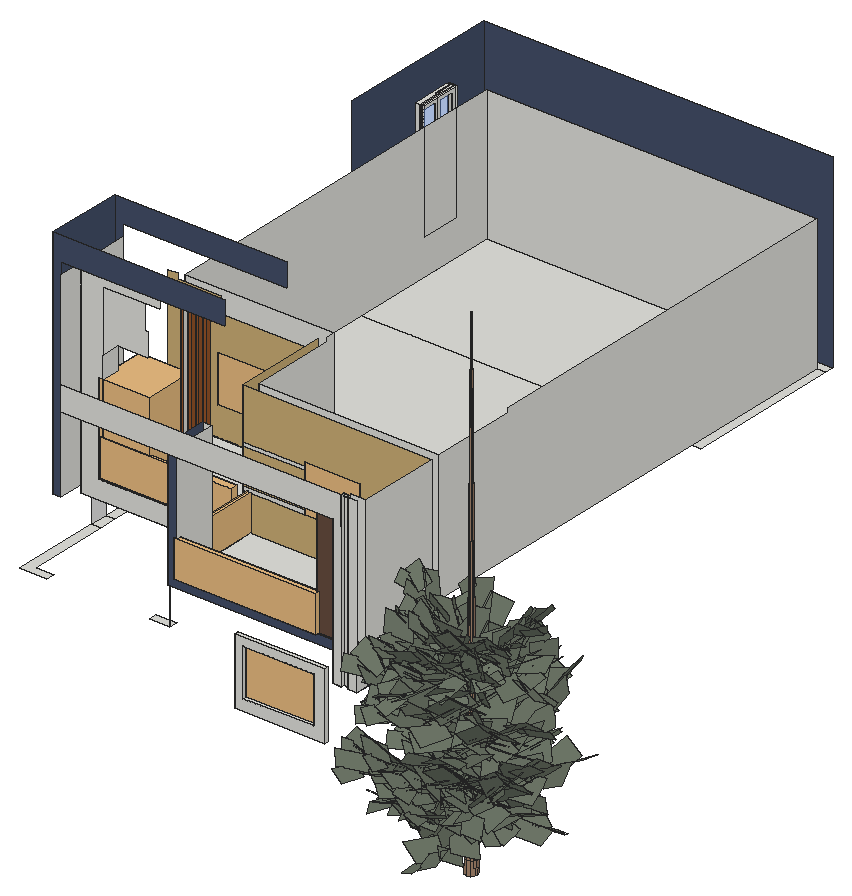
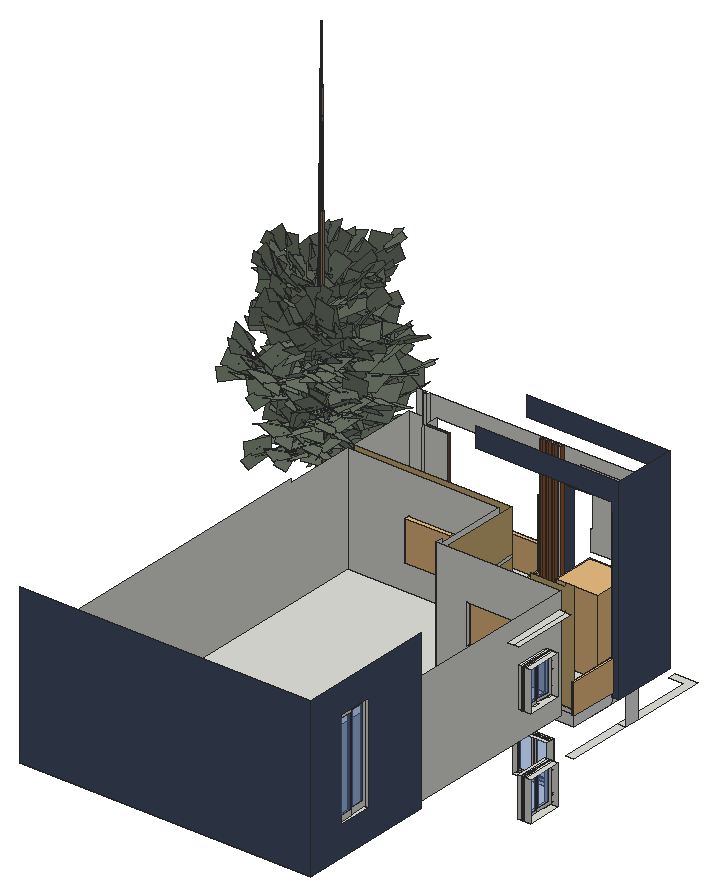
# SketchUp Ruby script. Lengths in inches.
U = 1.inch
M = Sketchup.active_model
def pt(a) = Geom::Point3d.new(a.map { |v| v * U })
def face(e, loops, mat)
  f = e.add_face(loops[0].map { |a| pt(a) })
  loops[1..].each { |l| e.add_face(l.map { |a| pt(a) }).erase! }
  f.material = f.back_material = mat if mat
  f
end
# faces: each face lists its corners as indices into pts; further lists are holes
def faces(e, pts, list, mat = nil) = list.each { |f| face(e, (f[0].is_a?(Array) ? f : [f]).map { |l| l.map { |i| pts[i] } }, mat) }
# xy, xz, yz: faces in a plane at the given z, y or x. An outline is a flat list of corners, or four numbers for a rectangle; further outlines are holes
def ring(l) = l.size == 4 ? [[l[0], l[1]], [l[2], l[1]], [l[2], l[3]], [l[0], l[3]]] : l.each_slice(2).to_a
def flat(e, list, mat, &to3) = list.each { |f| face(e, (f[0].is_a?(Array) ? f : [f]).map { |l| ring(l).map { |u, v| to3.(u, v) } }, mat) }
def xy(e, z, list, mat = nil) = flat(e, list, mat) { |x, y| [x, y, z] }
def xz(e, y, list, mat = nil) = flat(e, list, mat) { |x, z| [x, y, z] }
def yz(e, x, list, mat = nil) = flat(e, list, mat) { |y, z| [x, y, z] }
def lines(e, pts, list) = list.each { |a, b| e.add_line(pt(pts[a]), pt(pts[b])) }
# prism: a flat outline (further loops are holes) pulled along v
def prism(e, loops, v, mat = nil)
  f = face(e, loops, mat); d = Geom::Vector3d.new(v.map { |x| x * U })
  f.pushpull(f.normal.samedirection?(d) ? d.length : -d.length)
end
def box(e, o, s, mat = nil) = prism(e, [[o, [o[0] + s[0], o[1], o[2]], [o[0] + s[0], o[1] + s[1], o[2]], [o[0], o[1] + s[1], o[2]]]], [0, 0, s[2]], mat)
def at(x, y, z, deg = 0) = Geom::Transformation.translation(pt([x, y, z])) * Geom::Transformation.rotation(ORIGIN, Z_AXIS, deg.degrees)
def axes(o, x, y, z) = Geom::Transformation.new([*x, 0, *y, 0, *z, 0, *pt(o).to_a, 1])
def part(name) = M.definitions.add(name)
# library, detail: a bought-in or finely detailed component or shape, given as its bounding box
def library(name, o, s) = part(name).tap { |d| box(d.entities, o, s) }
def detail(e, o, s) = box(e.add_group.entities, o, s)
def put(e, d, t, mat = nil) = e.add_instance(d, t).tap { |i| i.material = mat if mat }
def group(e, t, mat = nil) = e.add_group.tap { |g| g.transformation = t; g.material = mat if mat }.entities
root = M.entities
M.materials.add("Marc_Shoes2").color = [68, 80, 105]
M.materials.add("Teddy_Glasses").color = [103, 77, 64]
M.materials.add("[Chipboard]").color = [205, 176, 119]
M.materials.add("[Translucent Glass Blue]").color = [100, 149, 237]
M.materials["[Translucent Glass Blue]"].alpha = 0.5
M.materials.add("[Wood Cherry Original]").color = [152, 86, 42]
M.materials.add("caule_pinheiro_fasdfa0d5asd9as0d15f9as16das5106w1560e1w6").color = [164, 132, 108]
M.materials.add("folha_pinheiro_fsadfaf0sa5f60a6s1d0fa19e01a601fw601").color = [111, 120, 105]
M.materials.add("white_wall").color = [233, 233, 233]
c1 = part("Janela aluminio")
xy(c1.entities,0,[[0,0,47.24,1.57],[23.62,1.57,47.24,2.76],[0,2.76,25.98,3.9375],[0,3.9375,47.24,5.91]])
xy(c1.entities,43.31,[[0,0,47.24,1.57],[23.62,1.57,47.24,2.76],[0,2.76,0,5.91,47.24,5.91,47.24,3.9375,25.98,3.9375,25.98,2.76],[25.98,2.76,47.24,3.9375]])
xz(c1.entities,1.57,[[0,0,23.62,0,23.62,41.34,21.26,41.34,21.26,1.97,1.97,1.97,1.97,41.34,23.62,41.34,23.62,43.31,0,43.31],[[23.62,0,47.24,43.31],[25.7,1.97,45.28,41.34]]])
xz(c1.entities,2.76,[[[0,0,23.62,43.31],[2.36,2.36,21.26,40.94]],[23.62,0,25.98,43.31]])
xz(c1.entities,2.76,[[2.36,2.36,21.26,40.94]],"[Translucent Glass Blue]")
xz(c1.entities,3.9375,[[25.98,0,25.98,2.36,44.88,2.36,44.88,40.94,25.98,40.94,25.98,43.31,47.24,43.31,47.24,0]])
xz(c1.entities,3.9375,[[25.98,2.36,44.88,40.94]],"[Translucent Glass Blue]")
yz(c1.entities,0,[[0,0,1.57,43.31],[2.76,0,5.91,43.31]])
yz(c1.entities,23.62,[[1.57,0,2.76,43.31]])
yz(c1.entities,25.98,[[2.76,0,3.9375,43.31]])
yz(c1.entities,47.24,[[0,0,1.57,43.31],[1.57,0,2.76,43.31],[3.9375,0,5.91,43.31]])
c2 = library("Janela+de+correr+1,50x1,00+m+VRAY",[0,0,0],[59.06,5.12,39.37])
c3 = part("bough01")
p = [[11.29,3.2,8.88],[13.41,4.42,-0.24],[13.19,18.86,1.64],[11.08,17.64,10.76],[8.3,5.16,4.77],[17.24,0,0],
  [26.01,15.19,0],[17.07,20.36,4.77],[7.28,2.65,0.91],[15.18,7.21,3.36],[7.9,19.82,3.36],[0,15.26,0.91],
  [8.87,11.62,4.48],[17.62,18.34,1.72],[8.85,32.26,7.82],[0.1,25.53,10.58],[10.83,18.83,5.84],[18.73,15.63,1.77],
  [26.01,27.18,6.84],[18.11,30.37,10.91],[8.25,26.54,5.5],[14.01,28.875,8.47],[10.03,38.73,8.47],[4.26,36.4,5.5],
  [10.04,24.31,6.06],[17.58,22.66,9.11],[19.2,35.07,11.83],[11.65,36.72,8.78]]
faces(c3.entities,p,[[0,1,2,3],[4,5,6,7],[8,9,10,11],[12,13,14,15],[16,17,18,19],[20,21,22,23],[24,25,26,27]],"folha_pinheiro_fsadfaf0sa5f60a6s1d0fa19e01a601fw601")
c4 = part("Group\#64")
put(c4.entities,c3,axes([22.61,-7.4375,0.27],[0.83269,0.71876,0],[-0.71876,0.83269,0],[0,0,1.1]))
put(c4.entities,c3,axes([17.06,9.8,0.27],[1.09059,0.14358,0],[-0.14358,1.09059,0],[0,0,1.1]))
c5 = library("Group\#23",[0,0,0],[144.29,5.15,36.98])
c6 = library("Group\#24",[0,0,0],[3.15,53.89,36.98])
c7 = library("Group\#27",[0,0,0],[3.15,61.52,36.98])
c8 = library("P1.FBX",[-25.82,-25.95,0],[51.65,51.91,92.04])
c9 = part("Group\#18")
box(c9.entities,[0,0,0],[3.8125,3.8125,204])
c10 = library("Group\#26",[0,0,0],[28.6875,7.08,39.72])
c11 = library("Group\#25",[0,0,0],[82.7,3.15,36.98])
xy(root,24.15,[[441.07,313.12,532.88,317.13]])
xy(root,36,[[449.71,313.12,521.71,325.52],[372.21,424.52,381.21,460.52],[245.65,505.52,287.65,514.52],[213.74,537.64,229.21,579.64]])
xy(root,72,[[219.74,317.12,247.49,317.12,247.49,325.52,229.21,325.52,229.21,408.6,219.74,408.6],[351.48,317.12,372.21,325.52],[219.74,408.6,229.21,426.23],[219.74,426.23,229.21,505.52]])
xy(root,84,[[449.71,313.12,521.71,325.52],[372.21,367.52,381.21,403.52],[372.21,424.52,381.21,460.52],[245.65,505.52,287.65,514.52],[310.83,505.52,352.83,514.52],
  [213.74,537.64,229.21,579.64]])
xy(root,89.8125,[[549.96,302.12,549.96,317.13,574.21,317.13,574.21,302.12,564.85,302.12,564.85,305.12,558.35,305.12,558.35,302.12],[558.35,302.12,558.74,305.12]])
xy(root,91.74,[[441.07,313.12,532.88,317.13]])
xy(root,106.875,[[219.74,457.52,372.21,505.52]])
xy(root,106.875,[[219.74,394.5,372.21,394.5,372.21,457.52,219.74,457.52,219.74,426.23,235.21,426.23,235.21,408.6,219.74,408.6]],"white_wall")
xy(root,111.01,[[372.21,315.12,549.96,317.13]])
xy(root,114,[[211.37,369.3125,211.37,447.9375,219.74,447.9375,219.74,426.23,214.46,426.23,214.46,408.6,219.74,408.6,219.74,369.3125],[214.46,408.6,219.74,426.23]],"Marc_Shoes2")
xy(root,120,[[381.21,315.12,381.21,409.52,565.21,409.52,565.21,325.52,549.96,325.52,549.96,321.32,521.53,321.32,521.53,315.12],[521.53,315.12,549.96,317.12],[372.21,359.56,381.21,409.52],[381.21,418.52,381.21,514.52,229.21,514.52,229.21,739.58,565.21,739.58,565.21,418.52],[219.74,739.58,219.74,907.52,574.21,907.52,574.21,898.52,229.21,898.52,229.21,739.58],
  [229.21,739.58,565.21,898.52],[565.21,739.58,574.21,898.52]])
xy(root,126,[[242.31,394.5,321.07,394.5,321.07,398.3125,324.88,398.3125,324.88,394.5,372.21,394.5,372.21,505.52,219.74,505.52,219.74,413.5625,242.31,413.5625],[321.07,394.5,324.88,398.3125]])
xy(root,156,[[435.96,409.52,491.34,418.52],[372.21,441.02,381.21,483.02],[270.21,505.52,343.34,514.52],[213.74,537.64,229.21,579.64],[229.21,537.64,258.43,579.64],
  [219.74,818.95,229.21,860.95]])
xy(root,204,[[435.96,409.52,491.34,418.52],[372.21,441.02,381.21,483.02],[270.21,505.52,343.34,514.52],[213.74,537.64,229.21,579.64],[229.21,537.64,258.43,579.64]])
xy(root,237.3,[[213.74,518.03,219.74,597.83],[219.74,518.03,227.09,597.83]])
xz(root,302.12,[[549.96,89.8125,558.74,89.8125,558.74,264.16,564.85,264.16,564.85,89.8125,574.21,89.8125,574.21,264.1875,272.99,264.1875,272.99,240,549.96,240]])
xz(root,305.12,[[558.74,89.8125,564.85,264.16]])
xz(root,313.12,[[[441.07,24.15,532.88,91.74],[449.71,36,521.71,84]]])
xz(root,315.12,[[372.21,111.01,549.96,111.01,549.96,120,381.21,120,381.21,240,372.21,240]],"Marc_Shoes2")
xz(root,317.12,[[521.53,120,549.96,240]],"Teddy_Glasses")
xz(root,321.32,[[521.53,120,549.96,240]])
xz(root,325.52,[[549.96,120,565.21,252]])
xz(root,359.56,[[372.21,120,381.21,240]])
xz(root,369.3125,[[211.37,114,219.74,114,219.74,328.22,386.12,328.22,386.12,352.25,211.37,352.25]],"Marc_Shoes2")
xz(root,394.5,[[219.74,106.875,372.21,106.875,372.21,126,242.31,126,242.31,302.34,300.31,302.34,300.31,316.1875,219.74,316.1875]])
xz(root,394.5,[[321.07,126,324.88,330]],"[Wood Cherry Original]")
xz(root,398.3125,[[321.07,126,324.88,330]])
xz(root,409.52,[[372.21,156.39,435.96,160.39],[372.21,196.61,435.96,200.61]])
xz(root,409.52,[[372.21,120,565.21,120,565.21,252,372.21,252,372.21,200.61,435.96,200.61,435.96,204,491.34,204,491.34,156,435.96,156,435.96,156.39,372.21,156.39],[372.21,160.39,435.96,196.61]],"[Chipboard]")
xz(root,413.5625,[[219.74,126,219.74,316.1875,300.31,316.1875,300.31,302.34,269.99,302.34,269.99,264.1875,272.99,264.1875,272.99,239.78,242.31,239.78,242.31,126]])
xz(root,418.52,[[[381.21,120,565.21,252],[435.96,156,491.34,204]]])
xz(root,424.52,[[372.21,36,381.21,84]])
xz(root,441.02,[[372.21,156,381.21,204]])
xz(root,447.9375,[[211.37,114,211.37,352.25,386.12,352.25,386.12,328.22,219.74,328.22,219.74,114]],"Marc_Shoes2")
xz(root,460.52,[[372.21,36,381.21,84]])
xz(root,483.02,[[372.21,156,381.21,204]])
xz(root,505.52,[[219.74,106.875,310.83,120],[310.83,106.875,372.21,120],[219.74,120,310.83,126],[310.83,120,372.21,126]])
xz(root,505.52,[[[219.74,126,372.21,126,372.21,240,272.99,240,272.99,256.375,229.21,256.375,229.21,261.3125,219.74,261.3125],[270.21,156,343.34,204]]],"[Chipboard]")
xz(root,514.52,[[[229.21,120,381.21,256.375],[270.21,156,343.34,204]]])
xz(root,537.64,[[213.74,36,229.21,84],[213.74,156,229.21,204],[229.21,156,258.43,204]])
xz(root,579.64,[[213.74,36,229.21,84],[213.74,156,229.21,204],[229.21,156,258.43,204]])
xz(root,818.95,[[219.74,156,229.21,276]])
xz(root,860.95,[[219.74,156,229.21,276]])
xz(root,898.52,[[229.21,120,565.21,256.375]])
xz(root,907.52,[[219.74,120,574.21,312]],"Marc_Shoes2")
yz(root,211.37,[[369.3125,114,447.9375,352.25]],"Marc_Shoes2")
yz(root,219.74,[[369.3125,114,394.5,316.1875],[394.5,114,447.9375,114,447.9375,126,413.5625,126,413.5625,316.1875,394.5,316.1875],[413.5625,126,447.9375,316.1875]])
yz(root,219.74,[[[739.58,120,907.52,312],[818.95,156,860.95,276]]],"Marc_Shoes2")
yz(root,219.74,[[408.6,72,426.23,114],[394.5,106.875,408.6,114],[426.23,106.875,447.9375,114],[447.9375,106.875,505.52,120],[447.9375,120,505.52,126]],"white_wall")
yz(root,229.21,[[[514.52,120,898.52,120,898.52,256.375,860.95,256.375,860.95,156,818.95,156,818.95,256.375,514.52,256.375],[537.64,156,579.64,204]],[818.95,156,860.95,256.375]])
yz(root,242.31,[[394.5,126,413.5625,239.78]])
yz(root,245.65,[[505.52,36,514.52,84]])
yz(root,258.43,[[537.64,156,579.64,204]])
yz(root,270.21,[[505.52,156,514.52,204]])
yz(root,287.65,[[505.52,36,514.52,84]])
yz(root,321.07,[[394.5,126,398.3125,330]],"[Wood Cherry Original]")
yz(root,324.88,[[394.5,126,398.3125,330]])
yz(root,343.34,[[505.52,156,514.52,204]])
yz(root,372.21,[[317.13,72,317.14,111.01,317.13,111.01],[317.13,72,317.14,72,317.14,111.01],[394.5,106.875,359.56,108.74,359.56,120,394.5,120],[394.5,106.875,409.52,120],[409.52,106.875,505.52,120],
  [394.5,120,409.52,126],[409.52,120,505.52,126],[441.02,155.18,409.52,156.39,409.52,160.39,441.02,159.18],[441.02,195.39,409.52,196.61,409.52,200.61,441.02,199.4]])
yz(root,372.21,[[359.56,108.74,317.14,111,317.14,111.01,315.12,111.01,315.12,240,359.56,240]],"Marc_Shoes2")
yz(root,372.21,[[409.52,126,409.52,156.39,441.02,155.18,441.02,156,483.02,156,483.02,204,441.02,204,441.02,199.4,409.52,200.61,409.52,252,505.52,252,505.52,126],[441.02,159.18,409.52,160.39,409.52,196.61,441.02,195.39]],"[Chipboard]")
yz(root,381.21,[[315.12,120,359.56,240],[[418.52,120,514.52,120,514.52,256.375,505.52,256.375,505.52,252,418.52,252],[441.02,156,483.02,204]]])
yz(root,435.96,[[409.52,156,418.52,204]])
yz(root,441.07,[[313.12,24.15,317.13,91.74]])
yz(root,449.71,[[313.12,36,325.52,84]])
yz(root,491.34,[[409.52,156,418.52,204]])
yz(root,521.53,[[317.12,120,321.32,240]],"Teddy_Glasses")
yz(root,521.71,[[313.12,36,325.52,84]])
yz(root,532.88,[[313.12,24.15,317.13,91.74]])
yz(root,549.96,[[302.12,89.8125,302.12,240,317.12,240,317.12,120,315.12,120,315.12,111.01,317.13,111.01,317.13,89.8125],[321.32,120,325.52,240]])
yz(root,558.35,[[305.12,89.8125,302.12,264.1875,306.12,264.26,309.12,89.88]])
yz(root,558.74,[[302.12,89.8125,305.12,264.16]])
yz(root,564.85,[[302.12,89.8125,305.12,264.16]])
yz(root,565.21,[[325.52,120,409.52,252],[418.52,120,418.52,252,505.52,252,505.52,256.375,898.52,256.375,898.52,120]])
yz(root,574.21,[[302.12,89.8125,325.52,120]])
p = [[558.74,305.12,89.8125],[558.35,305.12,89.8125],[558.35,309.12,89.88],[562.09,309.12,89.88],[562.09,305.12,89.8125],[562.09,306.12,264.26],
  [558.35,306.12,264.26],[372.21,325.52,120],[381.21,325.52,120],[219.74,518.03,240.39],[219.74,518.03,237.3]]
faces(root,p,[[0,1,2,3,4],[5,3,2,6]])
lines(root,p,[[7,8],[9,10]])
put(root,c1,axes([225.65,537.64,36],[0,0.889,0],[-1,0,0],[0,0,1.10836]))
put(root,c1,axes([378.12,424.52,36],[0,0.762,0],[-1,0,0],[0,0,1.10836]))
put(root,c2,axes([449.71,317.12,36],[1.22,0,0],[0,1,0],[0,0,1.2192]))
put(root,c1,axes([287.65,509.45,36],[-0.889,0,0],[0,-1,0],[0,0,1.10836]))
g1 = group(root,at(766.61,193.81,40.41))
xy(g1,0,[[6.18,0,3.09,0.83,0.83,3.09,0,6.18,0.83,9.27,3.09,11.53,6.18,12.36,9.27,11.53,11.53,9.27,12.36,6.18,11.53,3.09,9.27,0.83]])
xy(g1,510.44,[[6.18,5.65,6.45,5.72,6.64,5.91,6.71,6.18,6.64,6.45,6.45,6.64,6.18,6.71,5.91,6.64,5.72,6.45,5.65,6.18,5.72,5.91,5.91,5.72]])
p = [[6.18,0,0],[6.18,0.66,13.84],[3.42,1.4,13.84],[3.09,0.83,0],[9.27,0.83,0],[8.94,1.4,13.84],
  [1.4,3.42,13.84],[0.83,3.09,0],[11.53,3.09,0],[10.96,3.42,13.84],[0.66,6.18,13.84],[0,6.18,0],
  [12.36,6.18,0],[11.7,6.18,13.84],[1.4,8.94,13.84],[0.83,9.27,0],[11.53,9.27,0],[10.96,8.94,13.84],
  [3.42,10.96,13.84],[3.09,11.53,0],[9.27,11.53,0],[8.94,10.96,13.84],[6.18,11.7,13.84],[6.18,12.36,0],
  [6.18,2.37,95.48],[4.28,2.88,95.48],[8.08,2.88,95.48],[2.88,4.28,95.48],[9.48,4.28,95.48],[2.37,6.18,95.48],
  [9.99,6.18,95.48],[2.88,8.08,95.48],[9.48,8.08,95.48],[4.28,9.48,95.48],[8.08,9.48,95.48],[6.18,9.99,95.48],
  [6.18,5.65,510.44],[5.91,5.72,510.44],[6.45,5.72,510.44],[5.72,5.91,510.44],[6.64,5.91,510.44],[5.65,6.18,510.44],
  [6.71,6.18,510.44],[5.72,6.45,510.44],[6.64,6.45,510.44],[5.91,6.64,510.44],[6.45,6.64,510.44],[6.18,6.71,510.44]]
faces(g1,p,[[0,1,2,3],[4,5,1,0],[2,6,7,3],[8,9,5,4],[6,10,11,7],[9,8,12,13],[10,14,15,11],[13,12,16,17],
  [15,14,18,19],[17,16,20,21],[19,18,22,23],[23,22,21,20],[1,24,25,2],[5,26,24,1],[2,25,27,6],[9,28,26,5],
  [6,27,29,10],[9,13,30,28],[10,29,31,14],[13,17,32,30],[14,31,33,18],[17,21,34,32],[18,33,35,22],[22,35,34,21],
  [24,36,37,25],[26,38,36,24],[37,39,27,25],[28,40,38,26],[39,41,29,27],[28,30,42,40],[41,43,31,29],[30,32,44,42],
  [31,43,45,33],[32,34,46,44],[33,45,47,35],[35,47,46,34]],"caule_pinheiro_fasdfa0d5asd9as0d15f9as16das5106w1560e1w6")
put(root,c3,axes([769.57,223.85,96.37],[-0.26435,-2.09256,0],[-1.81221,0.22894,-1.0546],[-1.04628,0.13218,1.82662]))
put(root,c3,axes([754.91,215.92,97.72],[1.37819,-1.59665,0],[1.38274,1.19355,-1.0546],[0.79832,0.6891,1.82662]))
put(root,c3,axes([771.47,149.26,116.97],[0.24996,1.02803,-1.82466],[-2.08975,0.00096,-0.28573],[-0.13844,1.8417,1.01866]))
put(root,c3,axes([745.42,188.95,85.3],[2.06758,0.4169,0],[0.40269,-1.99713,-0.5459],[0.1079,-0.53513,2.03732]))
put(root,c3,axes([771.67,185.53,69.34],[0.26354,1.89925,0],[-1.52475,0.21158,1.14323],[1.13238,-0.15713,1.53936]))
put(root,c3,axes([771.73,143.14,115.22],[0.15447,2.10353,0],[-1.82171,0.13378,-1.0546],[-1.05176,0.07724,1.82662]))
put(root,c3,axes([778.16,210.18,75.59],[-0.82306,-0.98694,1.67249],[1.93704,-0.28773,0.78345],[-0.13844,1.8417,1.01866]))
put(root,c3,axes([765,198.3,75.59],[1.05603,-0.7323,1.67249],[0.11484,1.95492,0.78345],[-1.82217,-0.30119,1.01866]))
put(root,c3,axes([773.9,222.49,82.98],[-0.15447,-2.10353,0],[2.03185,-0.14921,0.5459],[-0.54443,0.03998,2.03732]))
put(root,c3,axes([789.65,199.19,82.98],[-2.10353,0.15447,0],[-0.14921,-2.03185,0.5459],[0.03998,0.54443,2.03732]))
put(root,c3,axes([781.27,186.49,82.98],[-1.37819,1.59665,0],[-1.54224,-1.33123,0.5459],[0.41324,0.3567,2.03732]))
put(root,c3,axes([750.5,201.27,82.97],[1.91745,0,0],[0,1.91745,0],[0,0,1.91745]))
put(root,c3,axes([789.41,177.8,90.36],[-1.1887,1.13286,0.99007],[-0.4286,-1.46449,1.16112],[1.44219,0.49852,1.16112]))
put(root,c3,axes([795.17,218.62,129.47],[-1.59665,-1.37819,0],[1.23976,-1.43628,-0.9213],[0.602,-0.69742,1.89734]))
put(root,c3,axes([756.55,209.62,96.55],[1.91745,0,0],[0,0.78601,1.74894],[0,-1.74894,0.78601]))
put(root,c4,axes([818.77,240.64,106.18],[-1.00393,-1.73187,0],[1.39934,-0.81117,1.17946],[-1.02041,0.59151,1.61745]))
put(root,c3,axes([756.67,188.33,100.43],[1.59665,1.37819,0],[-1.37819,1.59665,0],[0,0,2.10919]))
put(root,c4,axes([776.13,126.52,121.17],[-0.57172,1.53203,-0.32992],[-1.50467,-0.43845,0.57144],[0.43809,0.49343,1.53213]))
put(root,c3,axes([771.67,176.54,102.54],[0.26354,1.89925,0],[-1.52475,0.21158,1.14323],[1.13238,-0.15713,1.53936]))
put(root,c3,axes([774.73,190.58,108.76],[-0.27534,1.93295,0.79787],[-2.00262,-0.47541,0.46065],[0.602,-0.69742,1.89734]))
put(root,c4,axes([836.87,210.71,121.55],[-1.83938,-0.76286,0.20494],[0.78077,-1.67711,0.76483],[-0.11977,0.7827,1.83856]))
put(root,c4,axes([711.38,175.1,121.55],[1.76589,0.92027,0.20494],[-0.92397,1.60268,0.76483],[0.18753,-0.76928,1.83856]))
put(root,c4,axes([824.18,156.28,121.55],[-1.76188,0.92793,0.20494],[-0.79164,-1.67201,0.76483],[0.5257,0.59211,1.83856]))
g2 = group(root,at(701.49,190.23,116.66))
put(g2,c3,axes([52.03,-14.55,0.61],[1.91598,1.40575,0],[-1.65383,1.62858,0],[0,0,2.53103]))
put(g2,c3,axes([39.25,19.17,0.61],[2.50938,0.28081,0],[-0.33037,2.13297,0],[0,0,2.53103]))
put(root,c3,axes([754.44,181.84,117.72],[1.59665,1.37819,0],[1.37819,-1.59665,0],[0,0,2.10919]))
put(root,c5,at(379.23,313.55,120),"[Translucent Glass Blue]")
put(root,c6,at(377.3,357.59,120))
put(root,c7,at(218.17,445.97,120))
put(root,c4,axes([753.87,251.04,126.67],[0.95784,-2.0921,0],[1.72528,0.78989,0.21619],[-0.23683,-0.10843,2.28615]))
put(root,c4,axes([814.57,146.5625,126.74],[-1.49695,1.32906,0],[-1.32052,-1.48733,0.22661],[0.15045,0.16946,1.98895]))
put(root,c8,at(263.71,420.45,126))
put(root,c9,at(328.56,394.5,126),"[Wood Cherry Original]")
g3 = group(root,at(336.41,394.5,126),"[Wood Cherry Original]")
box(g3,[0,0,0],[3.8125,3.8125,204])
put(root,c9,at(343.97,394.5,126),"[Wood Cherry Original]")
put(root,c10,at(345.65,392.92,126))
put(root,c4,axes([744.93,255.76,136.32],[1.34596,-1.46754,0.20494],[1.0861,1.1654,1.21223],[-1.00799,-0.70387,1.5798]))
put(root,c11,at(240.34,392.92,128.54))
put(root,c4,axes([828.81,229.61,160.95],[-1.50227,-1.30708,0.20494],[1.27258,-1.3427,0.76483],[-0.36193,0.70425,1.83856]))
put(root,c4,axes([770.48,131.24,160.95],[-0.2194,1.97918,0.20494],[-1.82835,-0.28187,0.76483],[0.78504,-0.10335,1.83856]))
put(root,c2,axes([435.96,409.52,156],[0.93768,0,0],[0,3,0],[0,0,1.2192]))
put(root,c1,axes([229.21,818.95,156],[0,0.889,0],[-1.60308,0,0],[0,0,2.77091]))
put(root,c2,axes([270.21,505.52,156],[1.22,0,0],[0,1,0],[0,0,1.2192]))
put(root,c1,axes([225.65,537.64,156],[0,0.889,0],[-1,0,0],[0,0,1.10836]))
put(root,c1,axes([378.12,441.02,156],[0,0.889,0],[-1,0,0],[0,0,1.10836]))
put(root,c4,axes([750.4,128.43,156.06],[0.83208,2.14522,0],[-2.14522,0.83208,0],[0,0,2.30094]))
put(root,c3,axes([760.63,171.42,186.68],[1.11087,1.81277,0],[1.751,-1.07302,-0.69334],[0.46918,-0.28751,2.58757]))
put(root,c4,axes([834.4,217.13,166.15],[-1.78045,-0.91503,0],[0.90914,-1.769,0.22661],[-0.10358,0.20155,1.98895]))
put(root,c4,axes([715.02,198.66,166.11],[2.29689,0.13646,0],[-0.11525,1.93981,0.2214],[0.01545,-0.26002,2.28615]))
put(root,c4,axes([707.41,191.69,175.73],[1.85495,0.72417,0.20494],[-0.69377,1.43404,1.21223],[0.29172,-1.19432,1.5798]))
put(root,c3,axes([781.17,188.46,166.41],[-1.22158,1.4978,0],[-1.20246,-0.9807,1.45199],[0.89303,0.72834,1.95511]))
put(root,c3,axes([767.16,192.29,174.36],[1.26535,0.2773,2.1242],[-1.36472,1.4262,0.99505],[-1.02791,-1.55217,1.29378]))
put(root,c3,axes([767.42,210.16,174.36],[0.16401,-1.28495,2.1242],[1.54159,1.23288,0.99505],[-1.45491,1.16149,1.29378]))
put(root,c3,axes([751.43,213.2,221.3],[1.36377,-1.63104,0],[-1.41253,-1.18106,-1.06303],[-0.81552,-0.68188,1.84123]))
put(root,c3,axes([747.23,196.9375,222.66],[2.12464,-0.07791,0],[0.06747,1.83999,-1.06303],[0.03895,1.06232,1.84123]))
put(root,c3,axes([807.8125,163.42,242.07],[-0.58758,0.88997,-1.83926],[-1.43462,-1.54242,-0.28802],[-1.45491,1.16149,1.02681]))
put(root,c3,axes([755.41,215.46,183.73],[1.44726,-1.55744,0],[1.50437,1.39794,0.69334],[-0.40309,-0.37458,2.58757]))
put(root,c3,axes([783.42,211.11,183.73],[-1.55744,-1.44726,0],[1.39794,-1.50437,0.69334],[-0.37458,0.40309,2.58757]))
put(root,c3,axes([755.02,183.63,183.73],[1.31569,1.41585,0],[-1.41585,1.31569,0],[0,0,2.43531]))
put(root,c3,axes([794.62,198.15,189.53],[-1.37679,-0.08368,1.04789],[0.65608,-1.10113,1.22892],[0.51789,1.17248,1.22892]))
put(root,c3,axes([756.25,196.13,196.08],[1.09641,1.17988,0],[-0.48366,0.44944,1.85108],[1.07619,-1.00006,0.83191]))
put(root,c3,axes([772.86,228.51,242.79],[-0.07791,-2.12464,0],[1.91124,-0.07008,-1.17012],[0.92805,-0.03403,2.40978]))
put(root,c3,axes([812.51,159.41,240.3],[-1.44726,1.55744,0],[-1.34878,-1.25336,-1.06303],[-0.77872,-0.72363,1.84123]))
put(root,c3,axes([768.8125,179.3,205.9],[0.07791,2.12464,0],[-2.12464,0.07791,0],[0,0,2.67885]))
put(root,c3,axes([787.04,196.2,207.8],[-2.12464,0.07791,0],[-0.07525,-2.05224,0.55027],[0.02016,0.5499,2.05362]))
put(root,c3,axes([787.81,182.29,208.58],[-1.22158,1.4978,0],[-1.20246,-0.9807,1.45199],[0.89303,0.72834,1.95511]))
put(root,c4,axes([771.7,244.26,222.5],[0.40969,-1.34004,0],[1.08274,0.33103,1.04029],[-0.78955,-0.24139,1.42659]))
put(root,c3,axes([779.54,194.18,216.47],[-1.61623,1.12301,1.01336],[-1.02309,-1.80495,0.58506],[0.92805,-0.03403,2.40978]))
put(root,c4,axes([827.81,151.26,246.3],[-1.52355,0.62907,-0.33256],[-0.7087,-1.41191,0.57601],[-0.06375,0.66206,1.54439]))
put(root,c3,axes([772.08,173.2,227.85],[0.07791,2.12464,0],[2.12464,-0.07791,0],[0,0,2.67885]))
put(root,c4,axes([817.54,206.84,236.05],[-1.31537,-0.46129,0.18075],[0.48016,-1.20266,0.67458],[-0.05312,0.55171,1.62161]))
put(root,c4,axes([795.67,239.28,236.05],[-0.48529,-1.3067,0.18075],[1.23203,-0.39879,0.67458],[-0.45842,0.31154,1.62161]))
put(root,c4,axes([754.14,157.96,236.05],[0.36956,1.34403,0.18075],[-1.2621,0.28989,0.67458],[0.48383,-0.2704,1.62161]))
